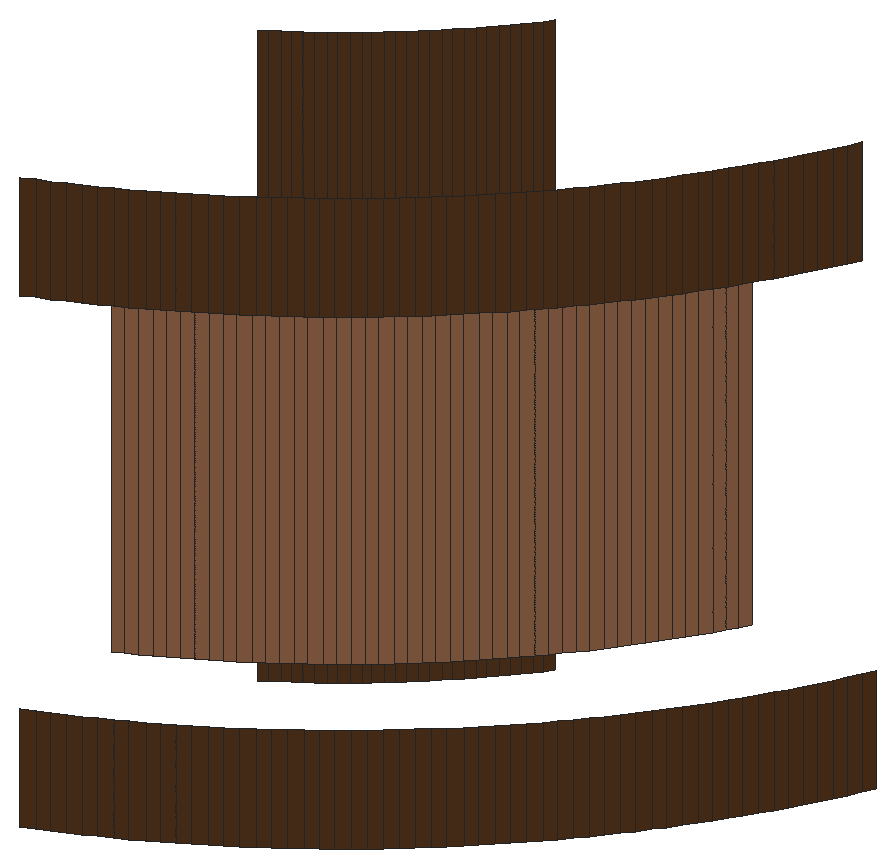
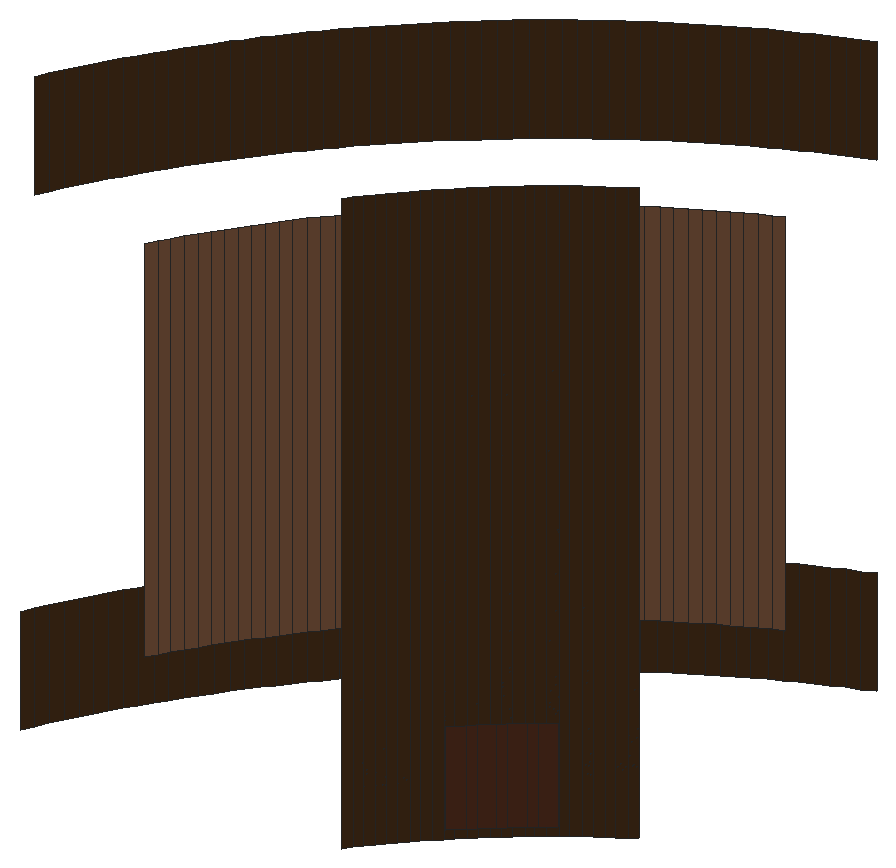
# SketchUp Ruby script. Lengths in inches.
U = 1.inch
M = Sketchup.active_model
def pt(a) = Geom::Point3d.new(a.map { |v| v * U })
def face(e, loops, mat)
  f = e.add_face(loops[0].map { |a| pt(a) })
  loops[1..].each { |l| e.add_face(l.map { |a| pt(a) }).erase! }
  f.material = f.back_material = mat if mat
  f
end
# faces: each face lists its corners as indices into pts; further lists are holes
def faces(e, pts, list, mat = nil) = list.each { |f| face(e, (f[0].is_a?(Array) ? f : [f]).map { |l| l.map { |i| pts[i] } }, mat) }
# xy, xz, yz: faces in a plane at the given z, y or x. An outline is a flat list of corners, or four numbers for a rectangle; further outlines are holes
def ring(l) = l.size == 4 ? [[l[0], l[1]], [l[2], l[1]], [l[2], l[3]], [l[0], l[3]]] : l.each_slice(2).to_a
def flat(e, list, mat, &to3) = list.each { |f| face(e, (f[0].is_a?(Array) ? f : [f]).map { |l| ring(l).map { |u, v| to3.(u, v) } }, mat) }
def xy(e, z, list, mat = nil) = flat(e, list, mat) { |x, y| [x, y, z] }
def xz(e, y, list, mat = nil) = flat(e, list, mat) { |x, z| [x, y, z] }
def yz(e, x, list, mat = nil) = flat(e, list, mat) { |y, z| [x, y, z] }
def lines(e, pts, list) = list.each { |a, b| e.add_line(pt(pts[a]), pt(pts[b])) }
# prism: a flat outline (further loops are holes) pulled along v
def prism(e, loops, v, mat = nil)
  f = face(e, loops, mat); d = Geom::Vector3d.new(v.map { |x| x * U })
  f.pushpull(f.normal.samedirection?(d) ? d.length : -d.length)
end
def box(e, o, s, mat = nil) = prism(e, [[o, [o[0] + s[0], o[1], o[2]], [o[0] + s[0], o[1] + s[1], o[2]], [o[0], o[1] + s[1], o[2]]]], [0, 0, s[2]], mat)
def at(x, y, z, deg = 0) = Geom::Transformation.translation(pt([x, y, z])) * Geom::Transformation.rotation(ORIGIN, Z_AXIS, deg.degrees)
def axes(o, x, y, z) = Geom::Transformation.new([*x, 0, *y, 0, *z, 0, *pt(o).to_a, 1])
def part(name) = M.definitions.add(name)
# library, detail: a bought-in or finely detailed component or shape, given as its bounding box
def library(name, o, s) = part(name).tap { |d| box(d.entities, o, s) }
def detail(e, o, s) = box(e.add_group.entities, o, s)
def put(e, d, t, mat = nil) = e.add_instance(d, t).tap { |i| i.material = mat if mat }
def group(e, t, mat = nil) = e.add_group.tap { |g| g.transformation = t; g.material = mat if mat }.entities
root = M.entities
M.materials.add("1799 AP 8574 BURNISHED CARAMEL").color = [140, 96, 69]
M.materials.add("1816 AP K197 Dark Kaapi-N").color = [79, 50, 27]
M.materials.add("[Wood Cherry Original]1").color = [93, 50, 33]
p = [[427.11,79.46,390],[427.32,79.56,390],[427.32,79.56,392],[427.11,79.46,392],[427.54,79.65,390],[427.54,79.65,392],
  [427.75,79.75,390],[427.75,79.75,392],[427.96,79.86,390],[427.96,79.86,392],[428.17,79.96,390],[428.17,79.96,392],
  [428.38,80.07,390],[428.38,80.07,392],[428.59,80.18,390],[428.59,80.18,392],[428.8,80.3,390],[428.8,80.3,392],
  [429,80.41,390],[429,80.41,392],[429.2,80.53,390],[429.2,80.53,392],[429.4,80.65,390],[429.4,80.65,392],
  [429.61,80.78,390],[429.61,80.78,392],[429.8,80.9,390],[429.8,80.9,392],[430,81.03,390],[430,81.03,392],
  [430.2,81.17,390],[430.2,81.17,392],[430.39,81.3,390],[430.39,81.3,392],[430.58,81.4375,390],[430.58,81.4375,392],
  [430.77,81.58,390],[430.77,81.58,392],[430.96,81.72,390],[430.96,81.72,392],[431.14,81.86,390],[431.14,81.86,392],
  [431.33,82.01,390],[431.33,82.01,392],[431.51,82.16,390],[431.51,82.16,392],[431.69,82.3125,390],[431.69,82.3125,392],
  [431.87,82.47,390],[431.87,82.47,392],[432.04,82.625,390],[432.04,82.625,392],[432.22,82.78,390],[432.22,82.78,392],
  [432.39,82.94,390],[432.39,82.94,392],[432.56,83.11,390],[432.56,83.11,392],[432.73,83.27,390],[432.73,83.27,392],
  [432.89,83.44,390],[432.89,83.44,392],[433.06,83.61,390],[433.06,83.61,392],[433.22,83.78,390],[433.22,83.78,392],
  [433.375,83.96,390],[433.375,83.96,392],[433.53,84.13,390],[433.53,84.13,392],[433.6875,84.31,390],[433.6875,84.31,392],
  [433.84,84.49,390],[433.84,84.49,392],[433.99,84.67,390],[433.99,84.67,392],[434.14,84.86,390],[434.14,84.86,392],
  [434.28,85.04,390],[434.28,85.04,392],[434.42,85.23,390],[434.42,85.23,392],[427.08,85.1,401],[427.22,85.19,401],
  [427.22,85.19,390],[427.08,85.1,390],[427.36,85.29,401],[427.36,85.29,390],[434.5625,85.42,390],[434.5625,85.42,392],
  [427.5,85.38,401],[427.5,85.38,390],[427.64,85.48,401],[427.64,85.48,390],[434.7,85.61,390],[434.7,85.61,392],
  [427.78,85.58,401],[427.78,85.58,390],[427.91,85.6875,401],[427.91,85.6875,390],[434.83,85.8,390],[434.83,85.8,392],
  [428.05,85.79,401],[428.05,85.79,390],[428.18,85.9,401],[428.18,85.9,390],[434.97,86,390],[434.97,86,392],
  [428.3125,86.01,401],[428.3125,86.01,390],[428.44,86.11,401],[428.44,86.11,390],[435.1,86.2,390],[435.1,86.2,392],
  [428.57,86.23,401],[428.57,86.23,390],[428.7,86.34,401],[428.7,86.34,390],[435.22,86.39,390],[435.22,86.39,392],
  [428.82,86.45,401],[428.82,86.45,390],[435.35,86.6,390],[435.35,86.6,392],[428.95,86.57,401],[428.95,86.57,390],
  [429.07,86.6875,401],[429.07,86.6875,390],[435.47,86.8,390],[435.47,86.8,392],[429.19,86.81,401],[429.19,86.81,390],
  [429.3125,86.93,401],[429.3125,86.93,390],[435.59,87,390],[435.59,87,392],[429.43,87.05,401],[429.43,87.05,390],
  [435.7,87.2,390],[435.7,87.2,392],[429.55,87.18,401],[429.55,87.18,390],[429.66,87.3,401],[429.66,87.3,390],
  [435.82,87.41,390],[435.82,87.41,392],[429.77,87.43,401],[429.77,87.43,390],[429.89,87.56,401],[429.89,87.56,390],
  [435.93,87.62,390],[435.93,87.62,392],[429.99,87.6875,401],[429.99,87.6875,390],[436.04,87.83,390],[436.04,87.83,392],
  [430.1,87.82,401],[430.1,87.82,390],[430.21,87.95,401],[430.21,87.95,390],[436.14,88.04,390],[436.14,88.04,392],
  [430.3125,88.09,401],[430.3125,88.09,390],[436.25,88.25,390],[436.25,88.25,392],[427.08,85.1,391],[427.22,85.19,391],
  [427.22,85.19,398],[427.08,85.1,398],[427.36,85.29,391],[427.36,85.29,398],[427.5,85.38,391],[427.5,85.38,398],
  [427.64,85.48,391],[427.64,85.48,398],[427.78,85.58,391],[427.78,85.58,398],[427.91,85.6875,391],[427.91,85.6875,398],
  [428.05,85.79,391],[428.05,85.79,398],[428.18,85.9,391],[428.18,85.9,398],[428.3125,86.01,391],[428.3125,86.01,398],
  [428.44,86.11,391],[428.44,86.11,398],[428.48,86.15,391],[428.57,86.23,391],[428.57,86.23,398],[428.7,86.34,391],
  [428.7,86.34,398],[428.82,86.45,391],[428.82,86.45,398],[428.95,86.57,391],[428.95,86.57,398],[429.07,86.6875,391],
  [429.07,86.6875,398],[429.19,86.81,391],[429.19,86.81,398],[429.3125,86.93,391],[429.3125,86.93,398],[429.43,87.05,391],
  [429.43,87.05,398],[427.35,87.16,391],[427.12,86.97,391],[427.12,86.97,392.75],[427.35,87.16,392.75],[429.55,87.18,391],
  [429.55,87.18,398],[427.47,87.26,391],[427.47,87.26,392.75],[429.66,87.3,391],[429.66,87.3,398],[427.69,87.45,391],
  [427.69,87.45,392.75],[429.77,87.43,391],[429.77,87.43,398],[429.89,87.56,391],[429.89,87.56,398],[427.81,87.56,391],
  [427.81,87.56,392.75],[428.02,87.76,391],[428.02,87.76,392.75],[429.99,87.6875,391],[429.99,87.6875,398],[430.1,87.82,391],
  [430.1,87.82,398],[428.13,87.87,391],[428.13,87.87,392.75],[430.21,87.95,391],[430.21,87.95,398],[428.34,88.08,391],
  [428.34,88.08,392.75],[430.3125,88.09,391],[430.3125,88.09,398],[427.08,81.65,392],[427.26,81.74,392],[427.26,81.74,399],
  [427.08,81.65,399],[427.45,81.84,392],[427.45,81.84,399],[427.63,81.9375,392],[427.63,81.9375,399],[427.82,82.04,392],
  [427.82,82.04,399],[428,82.14,392],[428,82.14,399],[428.18,82.25,392],[428.18,82.25,399],[428.36,82.36,392],
  [428.36,82.36,399],[428.54,82.47,392],[428.54,82.47,399],[428.71,82.58,392],[428.71,82.58,399],[428.89,82.7,392],
  [428.89,82.7,399],[429.0625,82.8125,392],[429.0625,82.8125,399],[429.23,82.93,392],[429.23,82.93,399],[429.4,83.06,392],
  [429.4,83.06,399],[429.57,83.18,392],[429.57,83.18,399],[429.74,83.31,392],[429.74,83.31,399],[429.91,83.43,392],
  [429.91,83.43,399],[430.07,83.57,392],[430.07,83.57,399],[430.23,83.7,392],[430.23,83.7,399],[430.39,83.83,392],
  [430.39,83.83,399],[430.55,83.97,392],[430.55,83.97,399],[430.71,84.11,392],[430.71,84.11,399],[430.86,84.25,392],
  [430.86,84.25,399],[431.01,84.39,392],[431.01,84.39,399],[431.16,84.54,392],[431.16,84.54,399],[431.3125,84.6875,392],
  [431.3125,84.6875,399],[431.46,84.84,392],[431.46,84.84,399],[431.61,84.99,392],[431.61,84.99,399],[431.75,85.14,392],
  [431.75,85.14,399],[431.89,85.29,392],[431.89,85.29,399],[432.03,85.45,392],[432.03,85.45,399],[432.17,85.61,392],
  [432.17,85.61,399],[432.3,85.77,392],[432.3,85.77,399],[432.43,85.93,392],[432.43,85.93,399],[432.57,86.09,392],
  [432.57,86.09,399],[432.69,86.26,392],[432.69,86.26,399],[432.82,86.43,392],[432.82,86.43,399],[432.94,86.6,392],
  [432.94,86.6,399],[433.07,86.77,392],[433.07,86.77,399],[433.1875,86.9375,392],[433.1875,86.9375,399],[433.3,87.11,392],
  [433.3,87.11,399],[433.42,87.29,392],[433.42,87.29,399],[433.53,87.46,392],[433.53,87.46,399],[433.64,87.64,392],
  [433.64,87.64,399],[433.75,87.82,392],[433.75,87.82,399],[433.86,88,392],[433.86,88,399],[433.96,88.18,392],
  [433.96,88.18,399],[427.11,79.46,399],[427.32,79.56,399],[427.32,79.56,401],[427.11,79.46,401],[427.54,79.65,399],
  [427.54,79.65,401],[427.75,79.75,399],[427.75,79.75,401],[427.96,79.86,399],[427.96,79.86,401],[428.17,79.96,399],
  [428.17,79.96,401],[428.38,80.07,399],[428.38,80.07,401],[428.59,80.18,399],[428.59,80.18,401],[428.8,80.3,399],
  [428.8,80.3,401],[429,80.41,399],[429,80.41,401],[429.2,80.53,399],[429.2,80.53,401],[429.4,80.65,399],
  [429.4,80.65,401],[429.61,80.78,399],[429.61,80.78,401],[429.8,80.9,399],[429.8,80.9,401],[430,81.03,399],
  [430,81.03,401],[430.2,81.17,399],[430.2,81.17,401],[430.39,81.3,399],[430.39,81.3,401],[430.58,81.4375,399],
  [430.58,81.4375,401],[430.77,81.58,399],[430.77,81.58,401],[430.96,81.72,399],[430.96,81.72,401],[431.14,81.86,399],
  [431.14,81.86,401],[431.33,82.01,399],[431.33,82.01,401],[431.51,82.16,399],[431.51,82.16,401],[431.69,82.3125,399],
  [431.69,82.3125,401],[431.87,82.47,399],[431.87,82.47,401],[432.04,82.625,399],[432.04,82.625,401],[432.22,82.78,399],
  [432.22,82.78,401],[432.39,82.94,399],[432.39,82.94,401],[432.56,83.11,399],[432.56,83.11,401],[432.73,83.27,399],
  [432.73,83.27,401],[432.89,83.44,399],[432.89,83.44,401],[433.06,83.61,399],[433.06,83.61,401],[433.22,83.78,399],
  [433.22,83.78,401],[433.375,83.96,399],[433.375,83.96,401],[433.53,84.13,399],[433.53,84.13,401],[433.6875,84.31,399],
  [433.6875,84.31,401],[433.84,84.49,399],[433.84,84.49,401],[433.99,84.67,399],[433.99,84.67,401],[434.14,84.86,399],
  [434.14,84.86,401],[434.28,85.04,399],[434.28,85.04,401],[434.42,85.23,399],[434.42,85.23,401],[434.5625,85.42,399],
  [434.5625,85.42,401],[434.7,85.61,399],[434.7,85.61,401],[434.83,85.8,399],[434.83,85.8,401],[434.97,86,399],
  [434.97,86,401],[435.1,86.2,399],[435.1,86.2,401],[435.22,86.39,399],[435.22,86.39,401],[435.35,86.6,399],
  [435.35,86.6,401],[435.47,86.8,399],[435.47,86.8,401],[435.59,87,399],[435.59,87,401],[435.7,87.2,399],
  [435.7,87.2,401],[435.82,87.41,399],[435.82,87.41,401],[435.93,87.62,399],[435.93,87.62,401],[436.04,87.83,399],
  [436.04,87.83,401],[436.14,88.04,399],[436.14,88.04,401],[428.48,84.5,391]]
faces(root,p,[[0,1,2,3],[1,4,5,2],[4,6,7,5],[6,8,9,7],[8,10,11,9],[10,12,13,11],[12,14,15,13],[14,16,17,15],
  [16,18,19,17],[18,20,21,19],[20,22,23,21],[22,24,25,23],[24,26,27,25],[26,28,29,27],[28,30,31,29],[30,32,33,31],
  [32,34,35,33],[34,36,37,35],[36,38,39,37],[38,40,41,39],[40,42,43,41],[42,44,45,43],[44,46,47,45],[46,48,49,47],
  [48,50,51,49],[50,52,53,51],[52,54,55,53],[54,56,57,55],[56,58,59,57],[58,60,61,59],[60,62,63,61],[62,64,65,63],
  [64,66,67,65],[66,68,69,67],[68,70,71,69],[70,72,73,71],[72,74,75,73],[74,76,77,75],[76,78,79,77],[78,80,81,79],
  [82,83,84,85],[83,86,87,84],[80,88,89,81],[86,90,91,87],[90,92,93,91],[88,94,95,89],[92,96,97,93],[96,98,99,97],
  [94,100,101,95],[98,102,103,99],[102,104,105,103],[100,106,107,101],[104,108,109,105],[108,110,111,109],[106,112,113,107],[110,114,115,111],
  [114,116,117,115],[112,118,119,113],[116,120,121,117],[118,122,123,119],[120,124,125,121],[124,126,127,125],[122,128,129,123],[126,130,131,127],
  [130,132,133,131],[128,134,135,129],[132,136,137,133],[134,138,139,135],[136,140,141,137],[140,142,143,141],[138,144,145,139],[142,146,147,143],
  [146,148,149,147],[144,150,151,145],[148,152,153,149],[150,154,155,151],[152,156,157,153],[156,158,159,157],[154,160,161,155],[158,162,163,159],
  [160,164,165,161],[331,332,333,334],[332,335,336,333],[335,337,338,336],[337,339,340,338],[339,341,342,340],[341,343,344,342],[343,345,346,344],
  [345,347,348,346],[347,349,350,348],[349,351,352,350],[351,353,354,352],[353,355,356,354],[355,357,358,356],[357,359,360,358],[359,361,362,360],
  [361,363,364,362],[363,365,366,364],[365,367,368,366],[367,369,370,368],[369,371,372,370],[371,373,374,372],[373,375,376,374],[375,377,378,376],
  [377,379,380,378],[379,381,382,380],[381,383,384,382],[383,385,386,384],[385,387,388,386],[387,389,390,388],[389,391,392,390],[391,393,394,392],
  [393,395,396,394],[395,397,398,396],[397,399,400,398],[399,401,402,400],[401,403,404,402],[403,405,406,404],[405,407,408,406],[407,409,410,408],
  [409,411,412,410],[411,413,414,412],[413,415,416,414],[415,417,418,416],[417,419,420,418],[419,421,422,420],[421,423,424,422],[423,425,426,424],
  [425,427,428,426],[427,429,430,428],[429,431,432,430],[431,433,434,432],[433,435,436,434],[435,437,438,436],[437,439,440,438]],"1816 AP K197 Dark Kaapi-N")
faces(root,p,[[166,167,168,169],[167,170,171,168],[170,172,173,171],[172,174,175,173],[174,176,177,175],[176,178,179,177],[178,180,181,179],[180,182,183,181],
  [182,184,185,183],[184,186,187,185],[186,188,189,190,187],[189,191,192,190],[191,193,194,192],[193,195,196,194],[195,197,198,196],[197,199,200,198],
  [199,201,202,200],[201,203,204,202],[205,206,207,208],[203,209,210,204],[211,205,208,212],[209,213,214,210],[215,211,212,216],[213,217,218,214],
  [217,219,220,218],[221,215,216,222],[223,221,222,224],[219,225,226,220],[225,227,228,226],[229,223,224,230],[227,231,232,228],[233,229,230,234],
  [231,235,236,232]],"[Wood Cherry Original]1")
faces(root,p,[[237,238,239,240],[238,241,242,239],[241,243,244,242],[243,245,246,244],[245,247,248,246],[247,249,250,248],[249,251,252,250],[251,253,254,252],
  [253,255,256,254],[255,257,258,256],[257,259,260,258],[259,261,262,260],[261,263,264,262],[263,265,266,264],[265,267,268,266],[267,269,270,268],
  [269,271,272,270],[271,273,274,272],[273,275,276,274],[275,277,278,276],[277,279,280,278],[279,281,282,280],[281,283,284,282],[283,285,286,284],
  [285,287,288,286],[287,289,290,288],[289,291,292,290],[291,293,294,292],[293,295,296,294],[295,297,298,296],[297,299,300,298],[299,301,302,300],
  [301,303,304,302],[303,305,306,304],[305,307,308,306],[307,309,310,308],[309,311,312,310],[311,313,314,312],[313,315,316,314],[315,317,318,316],
  [317,319,320,318],[319,321,322,320],[321,323,324,322],[323,325,326,324],[325,327,328,326],[327,329,330,328]],"1799 AP 8574 BURNISHED CARAMEL")
lines(root,p,[[188,441]])
